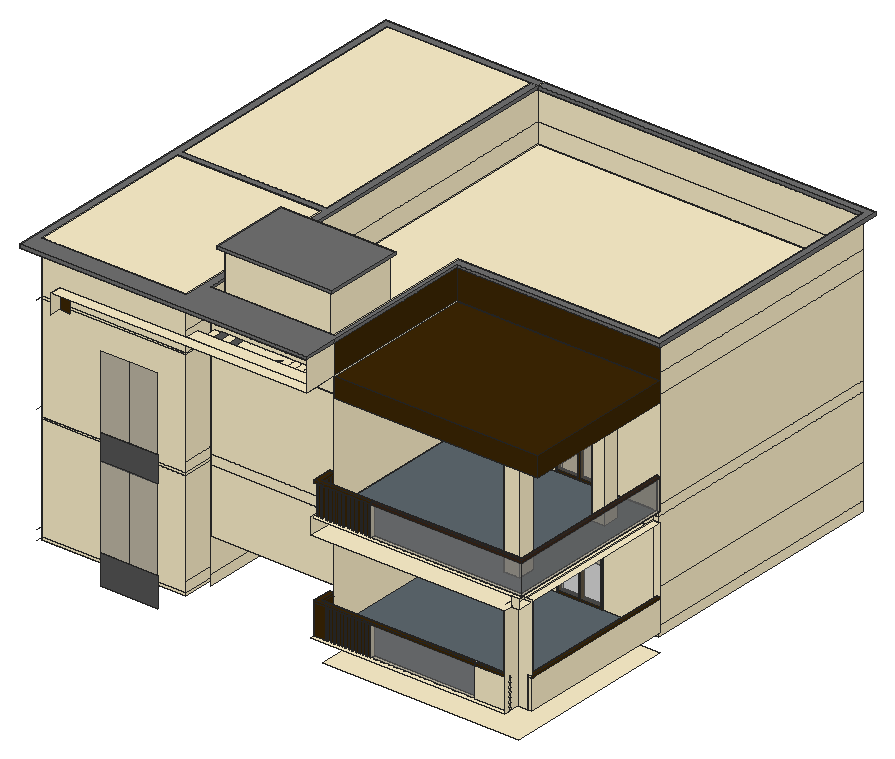
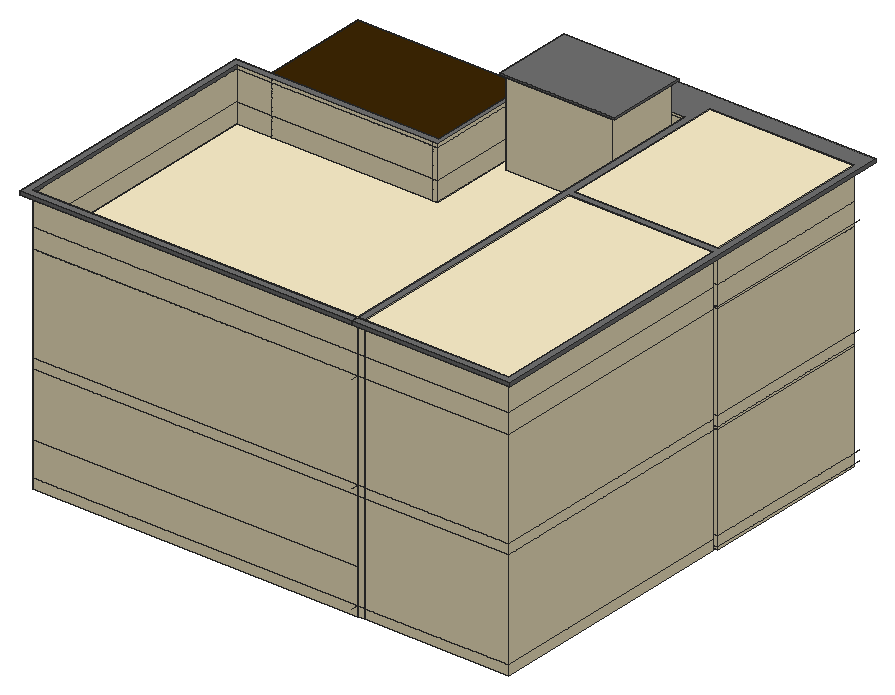
# SketchUp Ruby script. Lengths in inches.
U = 1.inch
M = Sketchup.active_model
def pt(a) = Geom::Point3d.new(a.map { |v| v * U })
def face(e, loops, mat)
  f = e.add_face(loops[0].map { |a| pt(a) })
  loops[1..].each { |l| e.add_face(l.map { |a| pt(a) }).erase! }
  f.material = f.back_material = mat if mat
  f
end
# faces: each face lists its corners as indices into pts; further lists are holes
def faces(e, pts, list, mat = nil) = list.each { |f| face(e, (f[0].is_a?(Array) ? f : [f]).map { |l| l.map { |i| pts[i] } }, mat) }
# xy, xz, yz: faces in a plane at the given z, y or x. An outline is a flat list of corners, or four numbers for a rectangle; further outlines are holes
def ring(l) = l.size == 4 ? [[l[0], l[1]], [l[2], l[1]], [l[2], l[3]], [l[0], l[3]]] : l.each_slice(2).to_a
def flat(e, list, mat, &to3) = list.each { |f| face(e, (f[0].is_a?(Array) ? f : [f]).map { |l| ring(l).map { |u, v| to3.(u, v) } }, mat) }
def xy(e, z, list, mat = nil) = flat(e, list, mat) { |x, y| [x, y, z] }
def xz(e, y, list, mat = nil) = flat(e, list, mat) { |x, z| [x, y, z] }
def yz(e, x, list, mat = nil) = flat(e, list, mat) { |y, z| [x, y, z] }
def lines(e, pts, list) = list.each { |a, b| e.add_line(pt(pts[a]), pt(pts[b])) }
# prism: a flat outline (further loops are holes) pulled along v
def prism(e, loops, v, mat = nil)
  f = face(e, loops, mat); d = Geom::Vector3d.new(v.map { |x| x * U })
  f.pushpull(f.normal.samedirection?(d) ? d.length : -d.length)
end
def box(e, o, s, mat = nil) = prism(e, [[o, [o[0] + s[0], o[1], o[2]], [o[0] + s[0], o[1] + s[1], o[2]], [o[0], o[1] + s[1], o[2]]]], [0, 0, s[2]], mat)
def at(x, y, z, deg = 0) = Geom::Transformation.translation(pt([x, y, z])) * Geom::Transformation.rotation(ORIGIN, Z_AXIS, deg.degrees)
def axes(o, x, y, z) = Geom::Transformation.new([*x, 0, *y, 0, *z, 0, *pt(o).to_a, 1])
def part(name) = M.definitions.add(name)
# library, detail: a bought-in or finely detailed component or shape, given as its bounding box
def library(name, o, s) = part(name).tap { |d| box(d.entities, o, s) }
def detail(e, o, s) = box(e.add_group.entities, o, s)
def put(e, d, t, mat = nil) = e.add_instance(d, t).tap { |i| i.material = mat if mat }
def group(e, t, mat = nil) = e.add_group.tap { |g| g.transformation = t; g.material = mat if mat }.entities
root = M.entities
M.materials.add("[Color C08]").color = [61, 39, 4]
M.materials.add("[Color C08]1").color = [60, 39, 24]
M.materials.add("[Color D01]").color = [255, 242, 204]
M.materials.add("[Color M05]").color = [114, 114, 114]
M.materials.add("[Color M06]").color = [86, 86, 86]
M.materials.add("[Formica Speckled Grey]").color = [94, 105, 111]
M.materials.add("[Translucent Glass Gray]").color = [128, 128, 128]
M.materials["[Translucent Glass Gray]"].alpha = 0.5
c1 = part("Group\#2")
xy(c1.entities,0,[[0,0,31.875,6]],"[Color C08]")
xy(c1.entities,1.18,[[1.18,0,15.1,6],[16.8,0,30.69,6]],"[Color C08]")
xy(c1.entities,43.63,[[1.18,0,15.1,6],[16.8,0,30.69,6]],"[Color C08]")
xy(c1.entities,44.8125,[[0,0,31.875,6]],"[Color C08]")
xz(c1.entities,0,[[[0,0,31.875,44.8125],[1.18,1.18,15.1,43.63],[16.8,1.18,30.69,43.63]]],"[Color C08]")
xz(c1.entities,0,[[1.18,1.18,15.1,43.63],[16.8,1.18,30.69,43.63]],"[Translucent Glass Gray]")
xz(c1.entities,6,[[[0,0,31.875,44.8125],[1.18,1.18,15.1,43.63],[16.8,1.18,30.69,43.63]]],"[Color C08]")
yz(c1.entities,0,[[0,0,6,44.8125]],"[Color C08]")
yz(c1.entities,1.18,[[0,1.18,6,43.63]],"[Color C08]")
yz(c1.entities,15.1,[[0,1.18,6,43.63]],"[Color C08]")
yz(c1.entities,16.8,[[0,1.18,6,43.63]],"[Color C08]")
yz(c1.entities,30.69,[[0,1.18,6,43.63]],"[Color C08]")
yz(c1.entities,31.875,[[0,0,6,44.8125]],"[Color C08]")
xy(root,241.4375,[[359.83,77.27,600,293.6875]],"[Color D01]")
xy(root,249,[[9,86.9375,184.87,293.6875]],"[Color D01]")
xy(root,252,[[9,86.9375,184.87,293.6875]],"[Color D01]")
xy(root,264,[[345.4375,77.27,583.3125,77.27,583.3125,82.27,413.33,82.27,413.33,86.27,410.9,86.27,410.9,82.27,409.02,82.27,409.02,86.27,406.58,86.27,406.58,82.27,404.71,82.27,404.71,86.27,402.27,86.27,402.27,82.27,400.4,82.27,400.4,86.27,397.96,86.27,397.96,82.27,396.08,82.27,396.08,86.27,393.65,86.27,393.65,82.27,391.77,82.27,391.77,86.27,389.33,86.27,389.33,82.27,387.46,82.27,387.46,86.27,385.02,86.27,385.02,82.27,383.15,82.27,383.15,86.27,380.71,86.27,380.71,82.27,378.83,82.27,378.83,86.27,376.4,86.27,376.4,82.27,374.52,82.27,374.52,86.27,372.08,86.27,372.08,82.27,370.21,82.27,370.21,86.27,367.77,86.27,367.77,82.27,365.9,82.27,365.9,86.27,363.46,86.27,363.46,82.27,361.58,82.27,361.58,86.27,359.83,86.27,359.83,82.27,345.4375,82.27],[345.4375,82.27,346.21,86.27],[346.21,82.27,346.21,86.27,345.4375,86.27,345.4375,105.9375,351.27,105.9375,351.27,86.27,352.96,86.27,352.96,82.27,350.52,82.27,350.52,86.27,348.65,86.27,348.65,82.27],[348.65,82.27,350.52,86.27],[352.96,82.27,354.83,86.27],
  [354.83,82.27,357.27,86.27],[357.27,82.27,359.15,86.27],[359.15,82.27,359.83,86.27],[415.21,82.27,583.3125,86.27],[596,96.83,600,293.6875]],"[Color D01]")
xy(root,264,[[[351.27,86.27,583.3125,86.27,583.3125,96.83,596,96.83,596,293.6875,529.33,293.6875,529.33,302.6875,473.39,302.6875,473.39,293.6875,351.27,293.6875],[555.58,109.65,575.02,130.09]]],"[Formica Speckled Grey]")
xy(root,300,[[359.83,82.27,361.58,86.27],[361.58,82.27,363.46,86.27],[363.46,82.27,365.9,86.27],[365.9,82.27,367.77,86.27],[367.77,82.27,370.21,86.27],
  [370.21,82.27,372.08,86.27],[372.08,82.27,374.52,86.27],[374.52,82.27,376.4,86.27],[376.4,82.27,378.83,86.27],[378.83,82.27,380.71,86.27],
  [380.71,82.27,383.15,86.27],[383.15,82.27,385.02,86.27],[385.02,82.27,387.46,86.27],[387.46,82.27,389.33,86.27],[389.33,82.27,391.77,86.27],
  [391.77,82.27,393.65,86.27],[393.65,82.27,396.08,86.27],[396.08,82.27,397.96,86.27],[397.96,82.27,400.4,86.27],[400.4,82.27,402.27,86.27],
  [402.27,82.27,404.71,86.27],[404.71,82.27,406.58,86.27],[406.58,82.27,409.02,86.27],[409.02,82.27,410.9,86.27],[410.9,82.27,413.33,86.27]])
xy(root,300,[[415.21,82.27,583.3125,86.27],[596,96.83,600,293.6875]],"[Color D01]")
xy(root,303,[[345.4375,82.27,415.21,82.27,415.21,86.27,351.27,86.27,351.27,105.9375,345.4375,105.9375],[415.21,82.27,541.93,86.27],[541.93,82.27,583.3125,86.27],[596,96.83,600,293.6875]],"[Color C08]")
xy(root,306,[[193.87,113.25,345.4375,113.25,345.4375,302.6875,591,302.6875,591,614.6875,193.87,614.6875]],"[Color D01]")
xy(root,348,[[473.39,293.6875,529.33,302.6875]],"[Color D01]")
xy(root,376.3125,[[345.64,77.27,345.64,105.9375,351.27,105.9375,351.27,293.6875,591,293.6875,591,96.83,583.3125,96.83,583.3125,77.27]],"[Color D01]")
xy(root,381,[[9,86.9375,184.87,293.6875]],"[Color D01]")
xy(root,384,[[591,77.27,600,293.6875],[9,86.9375,184.87,293.6875],[193.87,113.25,345.4375,113.25,345.4375,302.6875,591,302.6875,591,614.6875,193.87,614.6875]],"[Color D01]")
xy(root,396,[[345.64,77.27,345.64,105.9375,347.01,105.9375,347.01,102.85,351.27,102.85,351.27,99.125,347.01,99.125,347.01,96.04,351.27,96.04,351.27,92.25,347.01,92.25,347.01,89.17,351.27,89.17,351.27,86.27,348.86,86.27,348.86,82.27,351.33,82.27,351.33,86.27,354.3,86.27,354.3,82.27,356.77,82.27,356.77,86.27,359.61,86.27,359.61,82.27,362.08,82.27,362.08,86.27,364.92,86.27,364.92,82.27,367.4,82.27,367.4,86.27,370.24,86.27,370.24,82.27,372.71,82.27,372.71,86.27,375.55,86.27,375.55,82.27,378.02,82.27,378.02,86.27,380.86,86.27,380.86,82.27,383.33,82.27,383.33,86.27,386.17,86.27,386.17,82.27,388.65,82.27,388.65,86.27,391.49,86.27,391.49,82.27,393.96,82.27,393.96,86.27,396.8,86.27,396.8,82.27,399.27,82.27,399.27,86.27,402.11,86.27,402.11,82.27,404.58,82.27,404.58,86.27,407.42,86.27,407.42,82.27,409.9,82.27,409.9,86.27,412.74,86.27,412.74,82.27,600,82.27,600,77.27],[348.86,82.27,351.33,86.27],[354.3,82.27,356.77,86.27],[359.61,82.27,362.08,86.27],[364.92,82.27,367.4,86.27],
  [370.24,82.27,372.71,86.27],[375.55,82.27,378.02,86.27],[380.86,82.27,383.33,86.27],[386.17,82.27,388.65,86.27],[391.49,82.27,393.96,86.27],
  [396.8,82.27,399.27,86.27],[402.11,82.27,404.58,86.27],[407.42,82.27,409.9,86.27],[412.74,82.27,415.21,86.27],[415.21,82.27,415.21,86.27,596,86.27,596,293.6875,600,293.6875,600,82.27],
  [347.01,89.17,351.27,92.25],[347.01,96.04,351.27,99.125],[347.01,102.85,351.27,105.9375],[555.46,109.65,555.58,119.52],[555.46,119.52,555.58,130.09],
  [472.21,293.6875,529.33,302.6875]],"[Color D01]")
xy(root,396,[[[351.27,86.27,596,293.6875],[555.58,109.65,575.02,130.09],[559.33,239.98,575.02,258.73]]],"[Formica Speckled Grey]")
xy(root,431.9375,[[347.01,96.04,351.27,99.125]])
xy(root,432,[[345.64,82.27,345.64,105.9375,347.01,105.9375,347.01,102.85,351.27,102.85,351.27,92.25,347.01,92.25,347.01,89.17,351.27,89.17,351.27,86.27,348.86,86.27,348.86,82.27],[348.86,82.27,351.27,86.27],[351.27,82.27,351.33,86.27],[351.33,82.27,354.3,86.27],[354.3,82.27,356.77,86.27],
  [356.77,82.27,359.61,86.27],[359.61,82.27,362.08,86.27],[362.08,82.27,364.92,86.27],[364.92,82.27,367.4,86.27],[367.4,82.27,370.24,86.27],
  [370.24,82.27,372.71,86.27],[372.71,82.27,375.55,86.27],[375.55,82.27,378.02,86.27],[378.02,82.27,380.86,86.27],[380.86,82.27,383.33,86.27],
  [383.33,82.27,386.17,86.27],[386.17,82.27,388.65,86.27],[388.65,82.27,391.49,86.27],[391.49,82.27,393.96,86.27],[393.96,82.27,396.8,86.27],
  [396.8,82.27,399.27,86.27],[399.27,82.27,407.42,86.27],[407.42,82.27,409.9,86.27],[409.9,82.27,412.74,86.27],[415.21,82.27,415.21,86.27,596,86.27,596,293.6875,600,293.6875,600,82.27]],"[Color D01]")
xy(root,432.0625,[[402.11,82.27,404.58,86.27]],"[Color D01]")
xy(root,435,[[345.64,82.27,415.21,82.27,415.21,86.27,351.27,86.27,351.27,105.9375,345.64,105.9375]],"[Color C08]")
xy(root,435,[[415.21,82.27,600,82.27,600,293.6875,596,293.6875,596,86.27,415.21,86.27]],"[Color C08]1")
xy(root,480,[[472.21,293.6875,529.33,302.6875]],"[Color D01]")
xy(root,513,[[9,86.9375,184.87,293.6875]],"[Color D01]")
xy(root,516,[[[351.27,105.9375,600,293.6875],[559.33,239.98,575.02,258.73]]],"[Color C08]")
xy(root,516,[[9,86.9375,184.87,293.6875],[[193.87,113.25,345.4375,113.25,345.4375,302.6875,591,302.6875,591,614.6875,193.87,614.6875],[202.64,123.52,333.52,213.21]]],"[Color D01]")
xy(root,517.125,[[555.46,109.65,575.02,130.09]],"[Color D01]")
xy(root,540,[[351.27,105.9375,600,293.6875]],"[Color C08]")
xy(root,540,[[38.0625,63.84,351.27,77.27],[193.87,77.27,351.27,93.5625],[205.01,93.5625,213.95,105.9375],[222.89,93.5625,231.83,105.9375],[240.76,93.5625,240.76,105.9375,303.33,105.9375,303.33,94.125,312.26,94.125,312.26,105.9375,321.2,105.9375,321.2,94.125,330.14,94.125,330.14,105.9375,351.27,105.9375,351.27,93.5625],
  [303.33,94.125,312.26,105.9375],[321.2,94.125,330.14,105.9375]],"[Color D01]")
xy(root,540,[[213.95,93.5625,222.89,105.9375],[231.83,93.5625,240.76,105.9375],[249.7,94.125,258.64,105.9375],[267.58,94.125,276.51,105.9375],[285.45,94.125,294.39,105.9375],
  [303.33,94.125,312.26,105.9375],[321.2,94.125,330.14,105.9375]],"[Color M06]")
xy(root,576,[[0,63.84,0,623.6875,193.87,623.6875,193.87,614.6875,9,614.6875,9,302.6875,184.87,302.6875,184.87,614.6875,193.87,614.6875,193.87,113.25,345.4375,113.25,345.4375,302.6875,591,302.6875,591,614.6875,193.87,614.6875,193.87,623.6875,600,623.6875,600,293.6875,351.27,293.6875,351.27,105.9375,351.06,105.9375,351.06,63.84,9,63.84,9,86.9375,184.87,86.9375,184.87,293.6875,9,293.6875,9,63.84],[351.06,63.84,351.27,105.9375]],"[Color D01]")
xy(root,580,[[9,86.9375,184.87,293.6875],[9,302.6875,184.87,614.6875]],"[Color D01]")
xy(root,580,[[0,63.84,9,63.84,9,293.6875,184.87,293.6875,184.87,86.9375,9,86.9375,9,63.84,351.06,63.84,351.06,105.9375,351.27,105.9375,351.27,293.6875,600,293.6875,600,623.6875,193.87,623.6875,193.87,614.6875,591,614.6875,591,302.6875,345.4375,302.6875,345.4375,113.25,193.87,113.25,193.87,614.6875,184.87,614.6875,184.87,302.6875,9,302.6875,9,614.6875,193.87,614.6875,193.87,623.6875,0,623.6875]],"[Color M05]")
xy(root,620,[[202.64,123.52,333.52,213.21]],"[Color D01]")
xy(root,620,[[197.46,118.96,337.83,123.52],[197.46,123.52,202.64,216.34],[333.52,123.52,337.83,216.34],[202.64,213.21,333.52,216.34]],"[Color M05]")
xy(root,623,[[197.46,118.96,337.83,216.34]],"[Color M05]")
xz(root,63.84,[[0,576,351.06,580]],"[Color M05]")
xz(root,77.27,[[38.0625,516,51.05,540]],"[Color C08]")
xz(root,77.27,[[591,384,600,396]],"[Color D01]")
xz(root,77.27,[[88.18,230.37,158.54,266.14],[88.18,367.2,158.54,398.4]],"[Color M06]")
xz(root,77.27,[[88.18,266.14,123.36,367.2],[123.36,266.14,158.54,367.2],[88.18,398.4,123.36,488.21],[123.36,398.4,158.54,488.21]],"[Translucent Glass Gray]")
xz(root,82.27,[[345.4375,264,359.83,300],[361.58,264,363.46,300],[365.9,264,367.77,300],[370.21,264,372.08,300],[374.52,264,376.4,300],
  [378.83,264,380.71,300],[383.15,264,385.02,300],[387.46,264,389.33,300],[391.77,264,393.65,300],[396.08,264,397.96,300],
  [400.4,264,402.27,300],[404.71,264,406.58,300],[409.02,264,410.9,300],[413.33,264,415.21,300],[345.4375,300,359.83,303],
  [359.83,300,415.21,303],[415.21,300,541.93,303],[541.93,300,583.3125,303],[348.86,396,351.33,432],[354.3,396,356.77,432],
  [359.61,396,362.08,432],[364.92,396,367.4,432],[370.24,396,372.71,432],[375.55,396,378.02,432],[380.86,396,383.33,432],
  [386.17,396,388.65,432],[391.49,396,393.96,432],[396.8,396,399.27,432],[402.11,396,404.58,432],[407.42,396,409.9,432],
  [412.74,396,415.21,432],[345.64,432,402.11,432,402.11,432.0625,404.58,432.0625,404.58,432,415.21,432,415.21,435,345.64,435]],"[Color C08]")
xz(root,82.27,[[415.21,432,600,435]],"[Color C08]1")
xz(root,82.27,[[541.93,264,583.3125,300],[402.11,432,404.58,432.0625]],"[Color D01]")
xz(root,82.27,[[415.21,264,541.93,300],[415.21,396,600,432]],"[Translucent Glass Gray]")
xz(root,86.27,[[351.27,264,359.83,300],[361.58,264,363.46,300],[365.9,264,367.77,300],[370.21,264,372.08,300],[374.52,264,376.4,300],
  [378.83,264,380.71,300],[383.15,264,385.02,300],[387.46,264,389.33,300],[391.77,264,393.65,300],[396.08,264,397.96,300],
  [400.4,264,402.27,300],[404.71,264,406.58,300],[409.02,264,410.9,300],[413.33,264,415.21,300],[351.27,300,415.21,303],
  [415.21,300,541.93,303],[541.93,300,583.3125,303],[348.86,396,351.27,432],[354.3,396,356.77,432],[359.61,396,362.08,432],
  [364.92,396,367.4,432],[370.24,396,372.71,432],[375.55,396,378.02,432],[380.86,396,383.33,432],[386.17,396,388.65,432],
  [391.49,396,393.96,432],[396.8,396,399.27,432],[402.11,396,404.58,432],[407.42,396,409.9,432],[412.74,396,415.21,432],
  [351.27,432,351.27,435,415.21,435,415.21,432,404.58,432,404.58,432.0625,402.11,432.0625,402.11,432]],"[Color C08]")
xz(root,86.27,[[415.21,432,596,435]],"[Color C08]1")
xz(root,86.27,[[541.93,264,583.3125,300],[351.27,396,351.33,432],[402.11,432,404.58,432.0625]],"[Color D01]")
xz(root,86.27,[[415.21,264,541.93,300],[415.21,396,596,432]],"[Translucent Glass Gray]")
xz(root,86.9375,[[9,249,184.87,252],[9,252,184.87,381],[9,381,184.87,384],[9,384,184.87,513],[9,513,184.87,516],
  [9,516,184.87,576],[9,576,184.87,580]],"[Color D01]")
xz(root,89.17,[[347.01,396,351.27,432]],"[Color C08]")
xz(root,92.25,[[347.01,396,351.27,432]],"[Color C08]")
xz(root,96.04,[[347.01,396,351.27,431.9375]],"[Color C08]")
xz(root,96.83,[[583.3125,264,583.3125,376.3125,591,376.3125,591,385.9375,600,385.9375,600,303,596,303,596,264],[596,264,600,300],[596,300,600,303],[583.3125,376.3125,591,384]],"[Color D01]")
xz(root,99.125,[[347.01,396,351.27,431.9375]],"[Color C08]")
xz(root,102.85,[[347.01,396,351.27,432]],"[Color C08]")
xz(root,105.9375,[[351.27,516,600,540]],"[Color C08]")
xz(root,105.9375,[[345.4375,264,351.27,300],[345.4375,300,351.27,303],[345.64,376.3125,351.27,384],[345.4375,384,345.64,396],[345.64,384,351.27,396],
  [347.01,396,351.27,432],[345.64,432,351.27,435]],"[Color D01]")
xz(root,105.9375,[[351.06,576,351.27,580]],"[Color M05]")
xz(root,109.65,[[555.58,264,575.02,396],[555.46,396,575.02,517.125]],"[Color D01]")
xz(root,113.25,[[193.87,306,345.4375,384],[193.87,384,345.4375,396],[193.87,396,345.4375,516],[193.87,516,345.4375,540],[193.87,540,345.4375,576],
  [193.87,576,345.4375,580]],"[Color D01]")
xz(root,118.96,[[197.46,620,337.83,623]],"[Color M05]")
xz(root,123.52,[[202.64,516,333.52,620]],"[Color D01]")
xz(root,130.09,[[555.58,264,575.02,396],[555.46,396,575.02,517.125]],"[Color D01]")
xz(root,213.21,[[202.64,516,333.52,620]],"[Color D01]")
xz(root,216.34,[[197.46,620,337.83,623]],"[Color M05]")
xz(root,239.98,[[559.33,396,575.02,516]],"[Color D01]")
xz(root,258.73,[[559.33,396,575.02,516]],"[Color D01]")
xz(root,293.6875,[[351.27,540,600,576]],"[Color C08]")
xz(root,293.6875,[[9,249,184.87,252],[9,252,184.87,264],[9,264,184.87,381],[351.27,264,473.39,264,473.39,348,529.33,348,529.33,264,591,264,591,376.3125,351.27,376.3125],[591,264,596,264,596,303,600,303,600,384,591,384],
  [596,264,600,300],[596,300,600,303],[351.27,376.3125,591,396],[9,381,184.87,384],[9,384,184.87,396],
  [9,396,184.87,513],[351.27,396,472.21,396,472.21,480,529.33,480,529.33,396,596,396,596,435,600,435,600,516,351.27,516],[596,396,600,432],[596,432,600,435],[9,513,184.87,516],
  [9,516,184.87,540],[351.27,516,600,540],[9,540,184.87,576],[9,576,184.87,580]],"[Color D01]")
xz(root,293.6875,[[351.27,576,600,580]],"[Color M05]")
xz(root,302.6875,[[9,252,184.87,264],[345.4375,252,351.27,306],[351.27,252,351.27,306,473.39,306,473.39,264,529.33,264,529.33,306,591,306,591,252],[9,264,184.87,384],[345.4375,306,351.27,384],
  [351.27,306,351.27,384,548,384,548,306,529.33,306,529.33,348,473.39,348,473.39,306],[473.39,306,529.33,348],[548,306,591,384],[9,384,184.87,396],[345.4375,384,351.27,396],
  [351.27,384,548,396],[548,384,591,396],[9,396,184.87,516],[345.4375,396,351.27,516],[351.27,396,351.27,516,548,516,548,396,529.33,396,529.33,480,472.21,480,472.21,396],
  [472.21,396,529.33,480],[548,396,591,516],[9,516,184.87,540],[345.4375,516,351.27,540],[351.27,516,548,540],
  [548,516,591,540],[9,540,184.87,576],[345.4375,540,351.27,576],[351.27,540,548,576],[548,540,591,576],
  [9,576,184.87,580],[345.4375,576,351.27,580],[351.27,576,548,580],[548,576,591,580]],"[Color D01]")
xz(root,614.6875,[[9,252,184.87,264],[184.87,252,193.87,264],[193.87,252,591,264],[9,264,184.87,384],[184.87,264,193.87,384],
  [193.87,264,591,306],[193.87,306,591,384],[9,384,184.87,396],[184.87,384,193.87,396],[193.87,384,591,396],
  [9,396,184.87,516],[184.87,396,193.87,516],[193.87,396,591,516],[9,516,184.87,540],[184.87,516,193.87,540],
  [193.87,516,591,540],[9,540,184.87,576],[184.87,540,193.87,576],[193.87,540,591,576],[9,576,184.87,580],
  [184.87,576,193.87,580]],"[Color D01]")
xz(root,614.6875,[[193.87,576,591,580]],"[Color M05]")
xz(root,623.6875,[[0,576,193.87,580],[193.87,576,600,580]],"[Color M05]")
yz(root,0,[[63.84,576,623.6875,580]],"[Color M05]")
yz(root,9,[[86.9375,249,293.6875,252],[86.9375,252,293.6875,264],[302.6875,252,614.6875,264],[86.9375,264,293.6875,381],[302.6875,264,614.6875,384],
  [86.9375,381,293.6875,384],[86.9375,384,293.6875,396],[302.6875,384,614.6875,396],[86.9375,396,293.6875,513],[302.6875,396,614.6875,516],
  [86.9375,513,293.6875,516],[86.9375,516,293.6875,540],[302.6875,516,614.6875,540],[86.9375,540,293.6875,576],[302.6875,540,614.6875,576],
  [86.9375,576,293.6875,580],[302.6875,576,614.6875,580]],"[Color D01]")
yz(root,38.0625,[[63.84,516,77.27,540]],"[Color D01]")
yz(root,184.87,[[86.9375,249,293.6875,252],[86.9375,252,293.6875,264],[302.6875,252,614.6875,264],[86.9375,264,293.6875,381],[302.6875,264,614.6875,384],
  [86.9375,381,293.6875,384],[86.9375,384,293.6875,396],[302.6875,384,614.6875,396],[86.9375,396,293.6875,513],[302.6875,396,614.6875,516],
  [86.9375,513,293.6875,516],[86.9375,516,293.6875,540],[302.6875,516,614.6875,540],[86.9375,540,293.6875,576],[302.6875,540,614.6875,576],
  [86.9375,576,293.6875,580],[302.6875,576,614.6875,580]],"[Color D01]")
yz(root,193.87,[[113.25,252,614.6875,264],[113.25,264,614.6875,306],[113.25,306,614.6875,384],[113.25,384,614.6875,396],[113.25,396,614.6875,516],
  [113.25,516,614.6875,540],[113.25,540,614.6875,576],[614.6875,576,623.6875,580]],"[Color D01]")
yz(root,193.87,[[113.25,576,614.6875,580]],"[Color M05]")
yz(root,197.46,[[118.96,620,216.34,623]],"[Color M05]")
yz(root,202.64,[[123.52,516,213.21,620]],"[Color D01]")
yz(root,333.52,[[123.52,516,213.21,620]],"[Color D01]")
yz(root,337.83,[[118.96,620,216.34,623]],"[Color M05]")
yz(root,345.4375,[[82.27,300,105.9375,303]],"[Color C08]")
yz(root,345.4375,[[113.25,252,302.6875,306],[82.27,264,105.9375,300],[113.25,306,302.6875,384],[113.25,384,302.6875,396],[113.25,396,302.6875,516],
  [113.25,516,302.6875,540],[113.25,540,302.6875,576],[113.25,576,302.6875,580]],"[Color D01]")
yz(root,345.64,[[82.27,432,105.9375,435]],"[Color C08]")
yz(root,345.64,[[77.27,376.3125,105.9375,396]],"[Color D01]")
yz(root,347.01,[[89.17,396,92.25,432],[96.04,396,99.125,431.9375]],"[Color C08]")
yz(root,347.01,[[102.85,396,105.9375,432]],"[Color D01]")
yz(root,348.86,[[82.27,396,86.27,432]],"[Color C08]")
yz(root,351.06,[[63.84,576,105.9375,580]],"[Color M05]")
yz(root,351.27,[[86.27,264,105.9375,300],[86.27,300,105.9375,303],[89.17,396,92.25,432],[96.04,396,99.125,431.9375],[102.85,396,105.9375,432],
  [86.27,432,105.9375,435],[105.9375,540,293.6875,576]],"[Color C08]")
yz(root,351.27,[[105.9375,264,293.6875,376.3125],[105.9375,376.3125,293.6875,396],[105.9375,396,293.6875,516],[105.9375,516,293.6875,540],[63.84,540,105.9375,576]],"[Color D01]")
yz(root,351.27,[[105.9375,576,293.6875,580]],"[Color M05]")
yz(root,351.33,[[82.27,396,86.27,432]],"[Color C08]")
yz(root,354.3,[[82.27,396,86.27,432]],"[Color C08]")
yz(root,356.77,[[82.27,396,86.27,432]],"[Color C08]")
yz(root,359.61,[[82.27,396,86.27,432]],"[Color C08]")
yz(root,359.83,[[82.27,264,86.27,300]],"[Color C08]")
yz(root,361.58,[[82.27,264,86.27,300]],"[Color C08]")
yz(root,362.08,[[82.27,396,86.27,432]],"[Color C08]")
yz(root,363.46,[[82.27,264,86.27,300]],"[Color C08]")
yz(root,364.92,[[82.27,396,86.27,432]],"[Color C08]")
yz(root,365.9,[[82.27,264,86.27,300]],"[Color C08]")
yz(root,367.4,[[82.27,396,86.27,432]],"[Color C08]")
yz(root,367.77,[[82.27,264,86.27,300]],"[Color C08]")
yz(root,370.21,[[82.27,264,86.27,300]],"[Color C08]")
yz(root,370.24,[[82.27,396,86.27,432]],"[Color C08]")
yz(root,372.08,[[82.27,264,86.27,300]],"[Color C08]")
yz(root,372.71,[[82.27,396,86.27,432]],"[Color C08]")
yz(root,374.52,[[82.27,264,86.27,300]],"[Color C08]")
yz(root,375.55,[[82.27,396,86.27,432]],"[Color C08]")
yz(root,376.4,[[82.27,264,86.27,300]],"[Color C08]")
yz(root,378.02,[[82.27,396,86.27,432]],"[Color C08]")
yz(root,378.83,[[82.27,264,86.27,300]],"[Color C08]")
yz(root,380.71,[[82.27,264,86.27,300]],"[Color C08]")
yz(root,380.86,[[82.27,396,86.27,432]],"[Color C08]")
yz(root,383.15,[[82.27,264,86.27,300]],"[Color C08]")
yz(root,383.33,[[82.27,396,86.27,432]],"[Color C08]")
yz(root,385.02,[[82.27,264,86.27,300]],"[Color C08]")
yz(root,386.17,[[82.27,396,86.27,432]],"[Color C08]")
yz(root,387.46,[[82.27,264,86.27,300]],"[Color C08]")
yz(root,388.65,[[82.27,396,86.27,432]],"[Color C08]")
yz(root,389.33,[[82.27,264,86.27,300]],"[Color C08]")
yz(root,391.49,[[82.27,396,86.27,432]],"[Color C08]")
yz(root,391.77,[[82.27,264,86.27,300]],"[Color C08]")
yz(root,393.65,[[82.27,264,86.27,300]],"[Color C08]")
yz(root,393.96,[[82.27,396,86.27,432]],"[Color C08]")
yz(root,396.08,[[82.27,264,86.27,300]],"[Color C08]")
yz(root,396.8,[[82.27,396,86.27,432]],"[Color C08]")
yz(root,397.96,[[82.27,264,86.27,300]],"[Color C08]")
yz(root,399.27,[[82.27,396,86.27,432]],"[Color C08]")
yz(root,400.4,[[82.27,264,86.27,300]],"[Color C08]")
yz(root,402.11,[[82.27,396,86.27,432.0625]],"[Color C08]")
yz(root,402.27,[[82.27,264,86.27,300]],"[Color C08]")
yz(root,404.58,[[82.27,396,86.27,432.0625]],"[Color C08]")
yz(root,404.71,[[82.27,264,86.27,300]],"[Color C08]")
yz(root,406.58,[[82.27,264,86.27,300]],"[Color C08]")
yz(root,407.42,[[82.27,396,86.27,432]],"[Color C08]")
yz(root,409.02,[[82.27,264,86.27,300]],"[Color C08]")
yz(root,409.9,[[82.27,396,86.27,432]],"[Color C08]")
yz(root,410.9,[[82.27,264,86.27,300]],"[Color C08]")
yz(root,412.74,[[82.27,396,86.27,432]],"[Color C08]")
yz(root,413.33,[[82.27,264,86.27,300]],"[Color C08]")
yz(root,415.21,[[82.27,264,86.27,300],[82.27,396,86.27,432]],"[Color D01]")
yz(root,472.21,[[293.6875,396,302.6875,480]],"[Color D01]")
yz(root,473.39,[[293.6875,264,302.6875,348]],"[Color D01]")
yz(root,529.33,[[293.6875,264,302.6875,348],[293.6875,396,302.6875,480]],"[Color D01]")
yz(root,541.93,[[82.27,300,82.27,303,86.27,303]])
yz(root,555.46,[[109.65,396,130.09,517.125]],"[Color D01]")
yz(root,555.58,[[109.65,264,130.09,396]],"[Color D01]")
yz(root,559.33,[[239.98,396,258.73,516]],"[Color D01]")
yz(root,575.02,[[109.65,264,130.09,396],[109.65,396,130.09,517.125],[239.98,396,258.73,516]],"[Color D01]")
yz(root,583.3125,[[77.27,264,77.27,376.3125,96.83,376.3125,96.83,264,86.27,264,86.27,303,82.27,303,82.27,264],[82.27,264,86.27,300],[82.27,300,86.27,303]],"[Color D01]")
yz(root,591,[[302.6875,252,614.6875,264],[302.6875,264,614.6875,306],[302.6875,306,614.6875,384],[96.83,376.3125,293.6875,384],[77.27,384,96.83,385.9375],
  [302.6875,384,614.6875,396],[302.6875,396,614.6875,516],[302.6875,516,614.6875,540],[302.6875,540,614.6875,576]],"[Color D01]")
yz(root,591,[[302.6875,576,614.6875,580]],"[Color M05]")
yz(root,596,[[96.83,300,293.6875,303]],"[Color C08]")
yz(root,596,[[86.27,432,293.6875,435]],"[Color C08]1")
yz(root,596,[[96.83,264,293.6875,300]],"[Color D01]")
yz(root,596,[[86.27,396,293.6875,432]],"[Translucent Glass Gray]")
yz(root,600,[[96.83,300,293.6875,303],[105.9375,516,293.6875,540]],"[Color C08]")
yz(root,600,[[82.27,432,293.6875,435]],"[Color C08]1")
yz(root,600,[[96.83,264,293.6875,300]],"[Color D01]")
yz(root,600,[[293.6875,576,623.6875,580]],"[Color M05]")
yz(root,600,[[82.27,396,293.6875,432]],"[Translucent Glass Gray]")
p = [[9,86.9375,252],[9,77.27,252],[193.87,623.6875,264],[193.87,614.6875,264],[9,86.9375,264],[9,77.27,264],
  [193.87,623.6875,396],[193.87,614.6875,396],[9,86.9375,396],[9,77.27,396],[193.87,623.6875,516],[193.87,614.6875,516],
  [9,86.9375,516],[9,77.27,516],[583.3125,77.27,384],[583.3125,96.83,384],[541.93,86.27,264],[541.93,86.27,260.8125]]
lines(root,p,[[0,1],[2,3],[4,5],[6,7],[8,9],[10,11],[12,13],[14,15],[16,17]])
put(root,c1,axes([473.39,293.6875,263.34],[1.7549,0,0],[0,0.71875,0],[0,0,1.88924]))
put(root,c1,axes([472.21,293.6875,396],[1.79216,0,0],[0,0.71875,0],[0,0,1.87448]))
